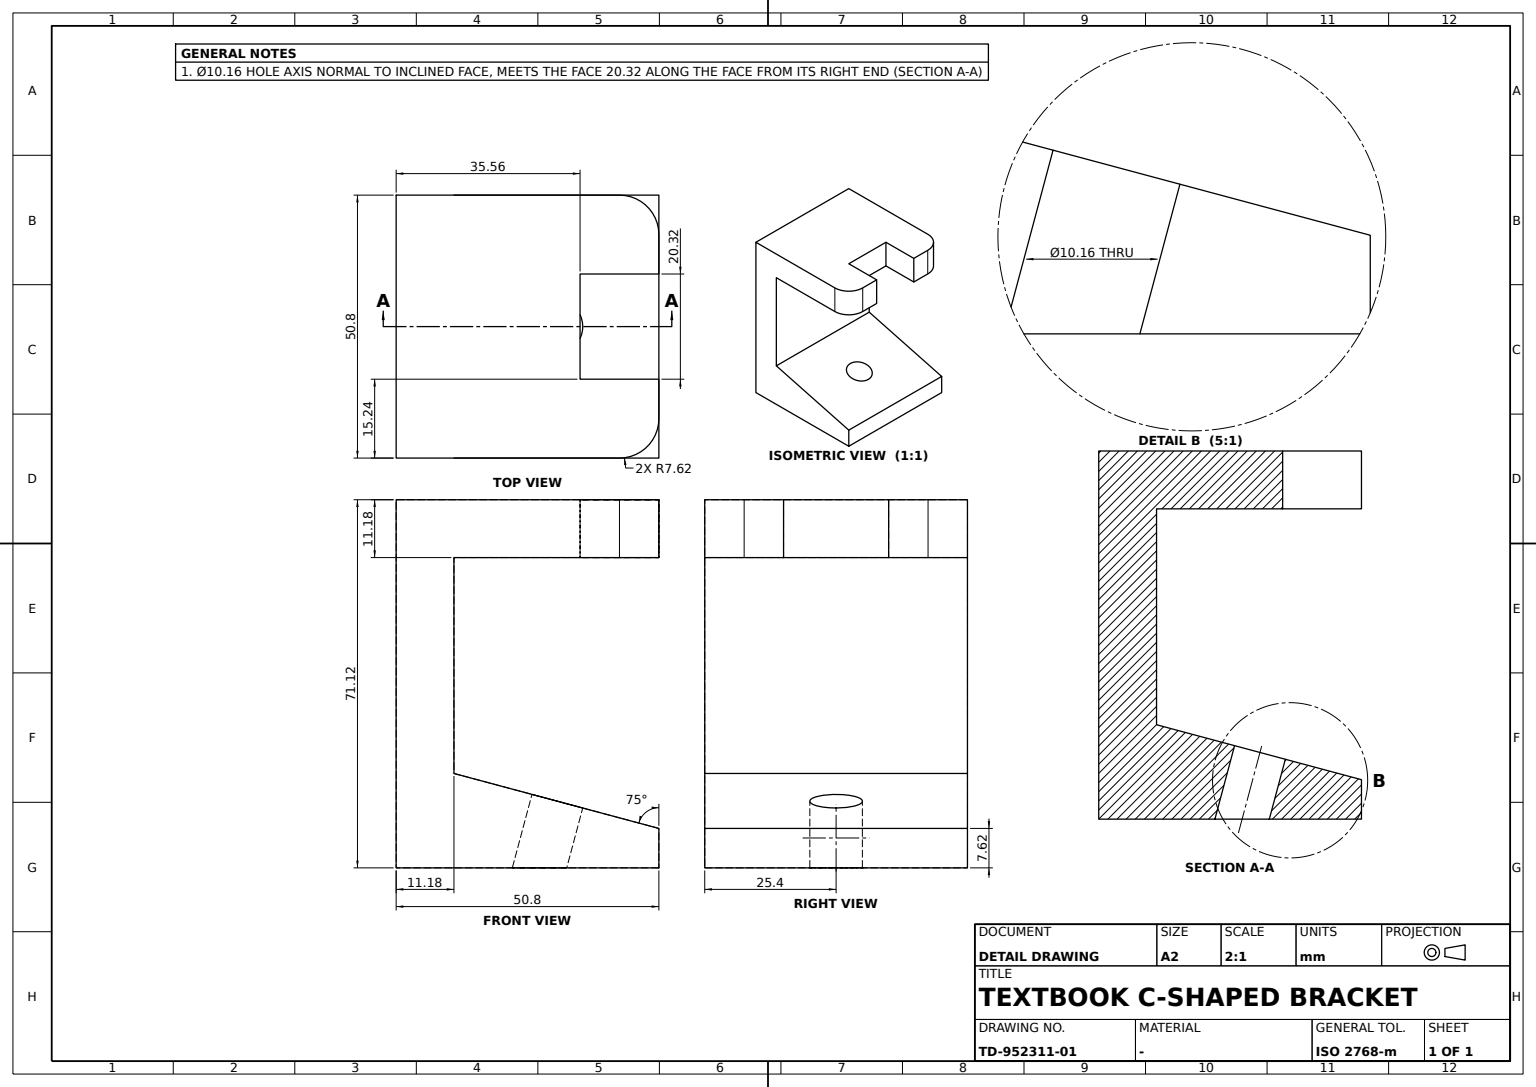
ISO-10303-21;
HEADER;
FILE_DESCRIPTION((''),'2;1');
FILE_NAME('','',(''),(''),'','','');
FILE_SCHEMA(('AUTOMOTIVE_DESIGN'));
ENDSEC;
DATA;
#1=APPLICATION_CONTEXT('');
#2=PRODUCT_CONTEXT('',#1,'mechanical');
#3=PRODUCT('','','',(#2));
#4=PRODUCT_DEFINITION_FORMATION('','',#3);
#5=PRODUCT_DEFINITION_CONTEXT('',#1,'design');
#6=PRODUCT_DEFINITION('','',#4,#5);
#7=PRODUCT_DEFINITION_SHAPE('','',#6);
#8=(LENGTH_UNIT()NAMED_UNIT(*)SI_UNIT(.MILLI.,.METRE.));
#9=(NAMED_UNIT(*)PLANE_ANGLE_UNIT()SI_UNIT($,.RADIAN.));
#10=(NAMED_UNIT(*)SI_UNIT($,.STERADIAN.)SOLID_ANGLE_UNIT());
#11=UNCERTAINTY_MEASURE_WITH_UNIT(LENGTH_MEASURE(0.005),#8,'distance_accuracy_value','');
#12=(GEOMETRIC_REPRESENTATION_CONTEXT(3)GLOBAL_UNCERTAINTY_ASSIGNED_CONTEXT((#11))GLOBAL_UNIT_ASSIGNED_CONTEXT((#8,#9,#10))REPRESENTATION_CONTEXT('',''));
#13=CARTESIAN_POINT('',(50.8,-17.78,71.12));
#14=VERTEX_POINT('',#13);
#15=CARTESIAN_POINT('',(50.8,-17.78,59.944));
#16=VERTEX_POINT('',#15);
#17=CARTESIAN_POINT('',(50.8,-17.78,35.56));
#18=DIRECTION('',(0.,0.,-1.));
#19=VECTOR('',#18,1000.);
#20=LINE('',#17,#19);
#21=EDGE_CURVE('',#14,#16,#20,.T.);
#22=ORIENTED_EDGE('',*,*,#21,.T.);
#23=CARTESIAN_POINT('',(50.8,-10.16,59.944));
#24=VERTEX_POINT('',#23);
#25=CARTESIAN_POINT('',(50.8,0.,59.944));
#26=DIRECTION('',(0.,1.,0.));
#27=VECTOR('',#26,1000.);
#28=LINE('',#25,#27);
#29=EDGE_CURVE('',#16,#24,#28,.T.);
#30=ORIENTED_EDGE('',*,*,#29,.T.);
#31=CARTESIAN_POINT('',(50.8,-10.16,71.12));
#32=VERTEX_POINT('',#31);
#33=LINE('',#31,#19);
#34=EDGE_CURVE('',#32,#24,#33,.T.);
#35=ORIENTED_EDGE('',*,*,#34,.F.);
#36=CARTESIAN_POINT('',(50.8,0.,71.12));
#37=LINE('',#36,#27);
#38=EDGE_CURVE('',#14,#32,#37,.T.);
#39=ORIENTED_EDGE('',*,*,#38,.F.);
#40=EDGE_LOOP('',(#22,#30,#35,#39));
#41=FACE_BOUND('',#40,.T.);
#42=DIRECTION('',(1.,0.,0.));
#43=AXIS2_PLACEMENT_3D('',#36,#42,#18);
#44=PLANE('',#43);
#45=ADVANCED_FACE('',(#41),#44,.T.);
#46=CARTESIAN_POINT('',(43.18,25.4,71.12));
#47=VERTEX_POINT('',#46);
#48=CARTESIAN_POINT('',(43.18,25.4,59.944));
#49=VERTEX_POINT('',#48);
#50=CARTESIAN_POINT('',(43.18,25.4,35.56));
#51=LINE('',#50,#19);
#52=EDGE_CURVE('',#47,#49,#51,.T.);
#53=ORIENTED_EDGE('',*,*,#52,.F.);
#54=CARTESIAN_POINT('',(50.8,17.78,71.12));
#55=VERTEX_POINT('',#54);
#56=CARTESIAN_POINT('',(43.18,17.78,71.12));
#57=DIRECTION('',(0.,0.,1.));
#58=AXIS2_PLACEMENT_3D('',#56,#57,#42);
#59=CIRCLE('',#58,7.62);
#60=EDGE_CURVE('',#55,#47,#59,.T.);
#61=ORIENTED_EDGE('',*,*,#60,.F.);
#62=CARTESIAN_POINT('',(50.8,17.78,59.944));
#63=VERTEX_POINT('',#62);
#64=CARTESIAN_POINT('',(50.8,17.78,35.56));
#65=LINE('',#64,#19);
#66=EDGE_CURVE('',#55,#63,#65,.T.);
#67=ORIENTED_EDGE('',*,*,#66,.T.);
#68=CARTESIAN_POINT('',(43.18,17.78,59.944));
#69=DIRECTION('',(-1.,0.,0.));
#70=AXIS2_PLACEMENT_3D('',#68,#18,#69);
#71=CIRCLE('',#70,7.62);
#72=EDGE_CURVE('',#49,#63,#71,.T.);
#73=ORIENTED_EDGE('',*,*,#72,.F.);
#74=EDGE_LOOP('',(#53,#61,#67,#73));
#75=FACE_BOUND('',#74,.T.);
#76=CARTESIAN_POINT('',(43.18,17.78,35.56));
#77=AXIS2_PLACEMENT_3D('',#76,#18,#42);
#78=CYLINDRICAL_SURFACE('',#77,7.62);
#79=ADVANCED_FACE('',(#75),#78,.T.);
#80=CARTESIAN_POINT('',(50.8,10.16,71.12));
#81=VERTEX_POINT('',#80);
#82=CARTESIAN_POINT('',(50.8,10.16,59.944));
#83=VERTEX_POINT('',#82);
#84=LINE('',#80,#19);
#85=EDGE_CURVE('',#81,#83,#84,.T.);
#86=ORIENTED_EDGE('',*,*,#85,.F.);
#87=CARTESIAN_POINT('',(35.56,10.16,71.12));
#88=VERTEX_POINT('',#87);
#89=VECTOR('',#42,1000.);
#90=LINE('',#87,#89);
#91=EDGE_CURVE('',#88,#81,#90,.T.);
#92=ORIENTED_EDGE('',*,*,#91,.F.);
#93=CARTESIAN_POINT('',(35.56,10.16,59.944));
#94=VERTEX_POINT('',#93);
#95=LINE('',#87,#19);
#96=EDGE_CURVE('',#88,#94,#95,.T.);
#97=ORIENTED_EDGE('',*,*,#96,.T.);
#98=VECTOR('',#69,1000.);
#99=LINE('',#93,#98);
#100=EDGE_CURVE('',#83,#94,#99,.T.);
#101=ORIENTED_EDGE('',*,*,#100,.F.);
#102=EDGE_LOOP('',(#86,#92,#97,#101));
#103=FACE_BOUND('',#102,.T.);
#104=AXIS2_PLACEMENT_3D('',#87,#26,#42);
#105=PLANE('',#104);
#106=ADVANCED_FACE('',(#103),#105,.F.);
#107=EDGE_CURVE('',#83,#63,#28,.T.);
#108=ORIENTED_EDGE('',*,*,#107,.F.);
#109=ORIENTED_EDGE('',*,*,#100,.T.);
#110=CARTESIAN_POINT('',(35.56,-10.16,59.944));
#111=VERTEX_POINT('',#110);
#112=CARTESIAN_POINT('',(35.56,0.,59.944));
#113=DIRECTION('',(0.,-1.,0.));
#114=VECTOR('',#113,1000.);
#115=LINE('',#112,#114);
#116=EDGE_CURVE('',#94,#111,#115,.T.);
#117=ORIENTED_EDGE('',*,*,#116,.T.);
#118=LINE('',#23,#98);
#119=EDGE_CURVE('',#24,#111,#118,.T.);
#120=ORIENTED_EDGE('',*,*,#119,.F.);
#121=ORIENTED_EDGE('',*,*,#29,.F.);
#122=CARTESIAN_POINT('',(43.18,-25.4,59.944));
#123=VERTEX_POINT('',#122);
#124=CARTESIAN_POINT('',(43.18,-17.78,59.944));
#125=AXIS2_PLACEMENT_3D('',#124,#18,#69);
#126=CIRCLE('',#125,7.62);
#127=EDGE_CURVE('',#16,#123,#126,.T.);
#128=ORIENTED_EDGE('',*,*,#127,.T.);
#129=CARTESIAN_POINT('',(11.176,-25.4,59.944));
#130=VERTEX_POINT('',#129);
#131=CARTESIAN_POINT('',(0.,-25.4,59.944));
#132=LINE('',#131,#98);
#133=EDGE_CURVE('',#123,#130,#132,.T.);
#134=ORIENTED_EDGE('',*,*,#133,.T.);
#135=CARTESIAN_POINT('',(11.176,25.4,59.944));
#136=VERTEX_POINT('',#135);
#137=CARTESIAN_POINT('',(11.176,0.,59.944));
#138=LINE('',#137,#27);
#139=EDGE_CURVE('',#130,#136,#138,.T.);
#140=ORIENTED_EDGE('',*,*,#139,.T.);
#141=CARTESIAN_POINT('',(0.,25.4,59.944));
#142=LINE('',#141,#98);
#143=EDGE_CURVE('',#49,#136,#142,.T.);
#144=ORIENTED_EDGE('',*,*,#143,.F.);
#145=ORIENTED_EDGE('',*,*,#72,.T.);
#146=EDGE_LOOP('',(#108,#109,#117,#120,#121,#128,#134,#140,#144,#145));
#147=FACE_BOUND('',#146,.T.);
#148=AXIS2_PLACEMENT_3D('',#25,#18,#69);
#149=PLANE('',#148);
#150=ADVANCED_FACE('',(#147),#149,.T.);
#151=CARTESIAN_POINT('',(43.18,-25.4,71.12));
#152=VERTEX_POINT('',#151);
#153=CARTESIAN_POINT('',(43.18,-17.78,71.12));
#154=AXIS2_PLACEMENT_3D('',#153,#57,#42);
#155=CIRCLE('',#154,7.62);
#156=EDGE_CURVE('',#152,#14,#155,.T.);
#157=ORIENTED_EDGE('',*,*,#156,.T.);
#158=ORIENTED_EDGE('',*,*,#38,.T.);
#159=CARTESIAN_POINT('',(35.56,-10.16,71.12));
#160=VERTEX_POINT('',#159);
#161=LINE('',#31,#98);
#162=EDGE_CURVE('',#32,#160,#161,.T.);
#163=ORIENTED_EDGE('',*,*,#162,.T.);
#164=LINE('',#87,#114);
#165=EDGE_CURVE('',#88,#160,#164,.T.);
#166=ORIENTED_EDGE('',*,*,#165,.F.);
#167=ORIENTED_EDGE('',*,*,#91,.T.);
#168=EDGE_CURVE('',#81,#55,#37,.T.);
#169=ORIENTED_EDGE('',*,*,#168,.T.);
#170=ORIENTED_EDGE('',*,*,#60,.T.);
#171=CARTESIAN_POINT('',(0.,25.4,71.12));
#172=VERTEX_POINT('',#171);
#173=LINE('',#171,#89);
#174=EDGE_CURVE('',#172,#47,#173,.T.);
#175=ORIENTED_EDGE('',*,*,#174,.F.);
#176=CARTESIAN_POINT('',(0.,-25.4,71.12));
#177=VERTEX_POINT('',#176);
#178=CARTESIAN_POINT('',(0.,0.,71.12));
#179=LINE('',#178,#27);
#180=EDGE_CURVE('',#177,#172,#179,.T.);
#181=ORIENTED_EDGE('',*,*,#180,.F.);
#182=LINE('',#176,#89);
#183=EDGE_CURVE('',#177,#152,#182,.T.);
#184=ORIENTED_EDGE('',*,*,#183,.T.);
#185=EDGE_LOOP('',(#157,#158,#163,#166,#167,#169,#170,#175,#181,#184));
#186=FACE_BOUND('',#185,.T.);
#187=AXIS2_PLACEMENT_3D('',#178,#57,#42);
#188=PLANE('',#187);
#189=ADVANCED_FACE('',(#186),#188,.T.);
#190=CARTESIAN_POINT('',(36.07929,0.,11.564402));
#191=VERTEX_POINT('',#190);
#192=CARTESIAN_POINT('',(31.172387,0.,12.879203));
#193=DIRECTION('',(0.258819045,0.,0.965925826));
#194=DIRECTION('',(0.965925826,0.,-0.258819045));
#195=AXIS2_PLACEMENT_3D('',#192,#193,#194);
#196=CIRCLE('',#195,5.08);
#197=EDGE_CURVE('',#191,#191,#196,.T.);
#198=ORIENTED_EDGE('',*,*,#197,.F.);
#199=EDGE_LOOP('',(#198));
#200=FACE_BOUND('',#199,.T.);
#201=CARTESIAN_POINT('',(11.176,25.4,18.237219));
#202=VERTEX_POINT('',#201);
#203=CARTESIAN_POINT('',(50.8,25.4,7.62));
#204=VERTEX_POINT('',#203);
#205=CARTESIAN_POINT('',(5.307955,25.4,19.809557));
#206=VECTOR('',#194,1000.);
#207=LINE('',#205,#206);
#208=EDGE_CURVE('',#202,#204,#207,.T.);
#209=ORIENTED_EDGE('',*,*,#208,.F.);
#210=CARTESIAN_POINT('',(11.176,-25.4,18.237219));
#211=VERTEX_POINT('',#210);
#212=CARTESIAN_POINT('',(11.176,0.,18.237219));
#213=LINE('',#212,#27);
#214=EDGE_CURVE('',#211,#202,#213,.T.);
#215=ORIENTED_EDGE('',*,*,#214,.F.);
#216=CARTESIAN_POINT('',(50.8,-25.4,7.62));
#217=VERTEX_POINT('',#216);
#218=CARTESIAN_POINT('',(5.307955,-25.4,19.809557));
#219=LINE('',#218,#206);
#220=EDGE_CURVE('',#211,#217,#219,.T.);
#221=ORIENTED_EDGE('',*,*,#220,.T.);
#222=CARTESIAN_POINT('',(50.8,0.,7.62));
#223=LINE('',#222,#27);
#224=EDGE_CURVE('',#217,#204,#223,.T.);
#225=ORIENTED_EDGE('',*,*,#224,.T.);
#226=EDGE_LOOP('',(#209,#215,#221,#225));
#227=FACE_BOUND('',#226,.T.);
#228=AXIS2_PLACEMENT_3D('',#212,#193,#194);
#229=PLANE('',#228);
#230=ADVANCED_FACE('',(#200,#227),#229,.T.);
#231=CARTESIAN_POINT('',(50.8,25.4,0.));
#232=VERTEX_POINT('',#231);
#233=LINE('',#231,#19);
#234=EDGE_CURVE('',#204,#232,#233,.T.);
#235=ORIENTED_EDGE('',*,*,#234,.F.);
#236=ORIENTED_EDGE('',*,*,#224,.F.);
#237=CARTESIAN_POINT('',(50.8,-25.4,0.));
#238=VERTEX_POINT('',#237);
#239=LINE('',#237,#19);
#240=EDGE_CURVE('',#217,#238,#239,.T.);
#241=ORIENTED_EDGE('',*,*,#240,.T.);
#242=CARTESIAN_POINT('',(50.8,0.,0.));
#243=LINE('',#242,#27);
#244=EDGE_CURVE('',#238,#232,#243,.T.);
#245=ORIENTED_EDGE('',*,*,#244,.T.);
#246=EDGE_LOOP('',(#235,#236,#241,#245));
#247=FACE_BOUND('',#246,.T.);
#248=ADVANCED_FACE('',(#247),#44,.T.);
#249=CARTESIAN_POINT('',(32.980618,0.,0.));
#250=VERTEX_POINT('',#249);
#251=CARTESIAN_POINT('',(27.721415,0.,0.));
#252=AXIS2_PLACEMENT_3D('',#251,#18,#42);
#253=ELLIPSE('',#252,5.259203,5.08);
#254=EDGE_CURVE('',#250,#250,#253,.F.);
#255=ORIENTED_EDGE('',*,*,#254,.T.);
#256=EDGE_LOOP('',(#255));
#257=FACE_BOUND('',#256,.T.);
#258=ORIENTED_EDGE('',*,*,#244,.F.);
#259=CARTESIAN_POINT('',(0.,-25.4,0.));
#260=VERTEX_POINT('',#259);
#261=LINE('',#259,#98);
#262=EDGE_CURVE('',#238,#260,#261,.T.);
#263=ORIENTED_EDGE('',*,*,#262,.T.);
#264=CARTESIAN_POINT('',(0.,25.4,0.));
#265=VERTEX_POINT('',#264);
#266=CARTESIAN_POINT('',(0.,0.,0.));
#267=LINE('',#266,#27);
#268=EDGE_CURVE('',#260,#265,#267,.T.);
#269=ORIENTED_EDGE('',*,*,#268,.T.);
#270=LINE('',#264,#98);
#271=EDGE_CURVE('',#232,#265,#270,.T.);
#272=ORIENTED_EDGE('',*,*,#271,.F.);
#273=EDGE_LOOP('',(#258,#263,#269,#272));
#274=FACE_BOUND('',#273,.T.);
#275=AXIS2_PLACEMENT_3D('',#242,#18,#69);
#276=PLANE('',#275);
#277=ADVANCED_FACE('',(#257,#274),#276,.T.);
#278=ORIENTED_EDGE('',*,*,#119,.T.);
#279=LINE('',#159,#19);
#280=EDGE_CURVE('',#160,#111,#279,.T.);
#281=ORIENTED_EDGE('',*,*,#280,.F.);
#282=ORIENTED_EDGE('',*,*,#162,.F.);
#283=ORIENTED_EDGE('',*,*,#34,.T.);
#284=EDGE_LOOP('',(#278,#281,#282,#283));
#285=FACE_BOUND('',#284,.T.);
#286=AXIS2_PLACEMENT_3D('',#31,#113,#69);
#287=PLANE('',#286);
#288=ADVANCED_FACE('',(#285),#287,.F.);
#289=ORIENTED_EDGE('',*,*,#96,.F.);
#290=ORIENTED_EDGE('',*,*,#165,.T.);
#291=ORIENTED_EDGE('',*,*,#280,.T.);
#292=ORIENTED_EDGE('',*,*,#116,.F.);
#293=EDGE_LOOP('',(#289,#290,#291,#292));
#294=FACE_BOUND('',#293,.T.);
#295=AXIS2_PLACEMENT_3D('',#87,#42,#113);
#296=PLANE('',#295);
#297=ADVANCED_FACE('',(#294),#296,.T.);
#298=ORIENTED_EDGE('',*,*,#220,.F.);
#299=CARTESIAN_POINT('',(11.176,-25.4,0.));
#300=LINE('',#299,#19);
#301=EDGE_CURVE('',#130,#211,#300,.T.);
#302=ORIENTED_EDGE('',*,*,#301,.F.);
#303=ORIENTED_EDGE('',*,*,#133,.F.);
#304=CARTESIAN_POINT('',(43.18,-25.4,35.56));
#305=LINE('',#304,#19);
#306=EDGE_CURVE('',#152,#123,#305,.T.);
#307=ORIENTED_EDGE('',*,*,#306,.F.);
#308=ORIENTED_EDGE('',*,*,#183,.F.);
#309=VECTOR('',#57,1000.);
#310=LINE('',#259,#309);
#311=EDGE_CURVE('',#260,#177,#310,.T.);
#312=ORIENTED_EDGE('',*,*,#311,.F.);
#313=ORIENTED_EDGE('',*,*,#262,.F.);
#314=ORIENTED_EDGE('',*,*,#240,.F.);
#315=EDGE_LOOP('',(#298,#302,#303,#307,#308,#312,#313,#314));
#316=FACE_BOUND('',#315,.T.);
#317=AXIS2_PLACEMENT_3D('',#259,#26,#69);
#318=PLANE('',#317);
#319=ADVANCED_FACE('',(#316),#318,.F.);
#320=LINE('',#264,#309);
#321=EDGE_CURVE('',#265,#172,#320,.T.);
#322=ORIENTED_EDGE('',*,*,#321,.F.);
#323=ORIENTED_EDGE('',*,*,#268,.F.);
#324=ORIENTED_EDGE('',*,*,#311,.T.);
#325=ORIENTED_EDGE('',*,*,#180,.T.);
#326=EDGE_LOOP('',(#322,#323,#324,#325));
#327=FACE_BOUND('',#326,.T.);
#328=AXIS2_PLACEMENT_3D('',#266,#69,#57);
#329=PLANE('',#328);
#330=ADVANCED_FACE('',(#327),#329,.T.);
#331=ORIENTED_EDGE('',*,*,#21,.F.);
#332=ORIENTED_EDGE('',*,*,#156,.F.);
#333=ORIENTED_EDGE('',*,*,#306,.T.);
#334=ORIENTED_EDGE('',*,*,#127,.F.);
#335=EDGE_LOOP('',(#331,#332,#333,#334));
#336=FACE_BOUND('',#335,.T.);
#337=CARTESIAN_POINT('',(43.18,-17.78,35.56));
#338=AXIS2_PLACEMENT_3D('',#337,#18,#113);
#339=CYLINDRICAL_SURFACE('',#338,7.62);
#340=ADVANCED_FACE('',(#336),#339,.T.);
#341=ORIENTED_EDGE('',*,*,#174,.T.);
#342=ORIENTED_EDGE('',*,*,#52,.T.);
#343=ORIENTED_EDGE('',*,*,#143,.T.);
#344=CARTESIAN_POINT('',(11.176,25.4,0.));
#345=LINE('',#344,#19);
#346=EDGE_CURVE('',#136,#202,#345,.T.);
#347=ORIENTED_EDGE('',*,*,#346,.T.);
#348=ORIENTED_EDGE('',*,*,#208,.T.);
#349=ORIENTED_EDGE('',*,*,#234,.T.);
#350=ORIENTED_EDGE('',*,*,#271,.T.);
#351=ORIENTED_EDGE('',*,*,#321,.T.);
#352=EDGE_LOOP('',(#341,#342,#343,#347,#348,#349,#350,#351));
#353=FACE_BOUND('',#352,.T.);
#354=AXIS2_PLACEMENT_3D('',#264,#26,#69);
#355=PLANE('',#354);
#356=ADVANCED_FACE('',(#353),#355,.T.);
#357=ORIENTED_EDGE('',*,*,#254,.F.);
#358=EDGE_LOOP('',(#357));
#359=FACE_BOUND('',#358,.T.);
#360=ORIENTED_EDGE('',*,*,#197,.T.);
#361=EDGE_LOOP('',(#360));
#362=FACE_BOUND('',#361,.T.);
#363=CARTESIAN_POINT('',(27.680882,0.,-0.151272));
#364=AXIS2_PLACEMENT_3D('',#363,#193,#26);
#365=CYLINDRICAL_SURFACE('',#364,5.08);
#366=ADVANCED_FACE('',(#359,#362),#365,.F.);
#367=ORIENTED_EDGE('',*,*,#346,.F.);
#368=ORIENTED_EDGE('',*,*,#139,.F.);
#369=ORIENTED_EDGE('',*,*,#301,.T.);
#370=ORIENTED_EDGE('',*,*,#214,.T.);
#371=EDGE_LOOP('',(#367,#368,#369,#370));
#372=FACE_BOUND('',#371,.T.);
#373=AXIS2_PLACEMENT_3D('',#137,#42,#18);
#374=PLANE('',#373);
#375=ADVANCED_FACE('',(#372),#374,.T.);
#376=ORIENTED_EDGE('',*,*,#85,.T.);
#377=ORIENTED_EDGE('',*,*,#107,.T.);
#378=ORIENTED_EDGE('',*,*,#66,.F.);
#379=ORIENTED_EDGE('',*,*,#168,.F.);
#380=EDGE_LOOP('',(#376,#377,#378,#379));
#381=FACE_BOUND('',#380,.T.);
#382=ADVANCED_FACE('',(#381),#44,.T.);
#383=CLOSED_SHELL('',(#45,#79,#106,#150,#189,#230,#248,#277,#288,#297,#319,#330,#340,#356,#366,#375,#382));
#384=MANIFOLD_SOLID_BREP('',#383);
#385=ADVANCED_BREP_SHAPE_REPRESENTATION('',(#384),#12);
#386=SHAPE_DEFINITION_REPRESENTATION(#7,#385);
ENDSEC;
END-ISO-10303-21;
